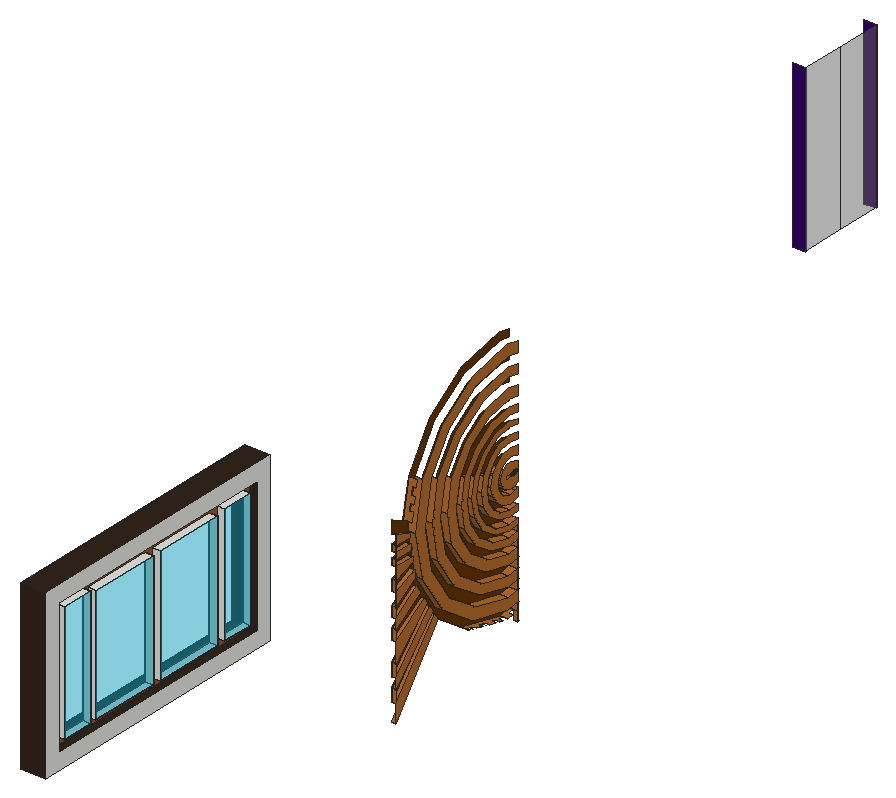
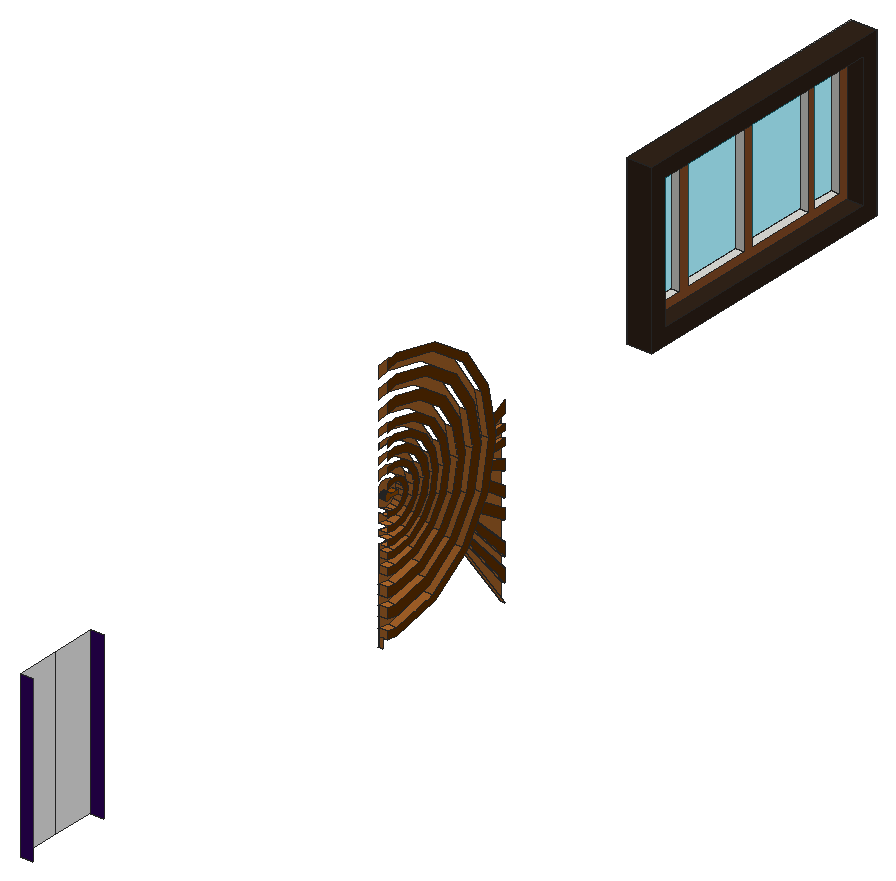
# SketchUp Ruby script. Lengths in inches.
U = 1.inch
M = Sketchup.active_model
def pt(a) = Geom::Point3d.new(a.map { |v| v * U })
def face(e, loops, mat)
  f = e.add_face(loops[0].map { |a| pt(a) })
  loops[1..].each { |l| e.add_face(l.map { |a| pt(a) }).erase! }
  f.material = f.back_material = mat if mat
  f
end
# faces: each face lists its corners as indices into pts; further lists are holes
def faces(e, pts, list, mat = nil) = list.each { |f| face(e, (f[0].is_a?(Array) ? f : [f]).map { |l| l.map { |i| pts[i] } }, mat) }
# xy, xz, yz: faces in a plane at the given z, y or x. An outline is a flat list of corners, or four numbers for a rectangle; further outlines are holes
def ring(l) = l.size == 4 ? [[l[0], l[1]], [l[2], l[1]], [l[2], l[3]], [l[0], l[3]]] : l.each_slice(2).to_a
def flat(e, list, mat, &to3) = list.each { |f| face(e, (f[0].is_a?(Array) ? f : [f]).map { |l| ring(l).map { |u, v| to3.(u, v) } }, mat) }
def xy(e, z, list, mat = nil) = flat(e, list, mat) { |x, y| [x, y, z] }
def xz(e, y, list, mat = nil) = flat(e, list, mat) { |x, z| [x, y, z] }
def yz(e, x, list, mat = nil) = flat(e, list, mat) { |y, z| [x, y, z] }
def lines(e, pts, list) = list.each { |a, b| e.add_line(pt(pts[a]), pt(pts[b])) }
# prism: a flat outline (further loops are holes) pulled along v
def prism(e, loops, v, mat = nil)
  f = face(e, loops, mat); d = Geom::Vector3d.new(v.map { |x| x * U })
  f.pushpull(f.normal.samedirection?(d) ? d.length : -d.length)
end
def box(e, o, s, mat = nil) = prism(e, [[o, [o[0] + s[0], o[1], o[2]], [o[0] + s[0], o[1] + s[1], o[2]], [o[0], o[1] + s[1], o[2]]]], [0, 0, s[2]], mat)
def at(x, y, z, deg = 0) = Geom::Transformation.translation(pt([x, y, z])) * Geom::Transformation.rotation(ORIGIN, Z_AXIS, deg.degrees)
def axes(o, x, y, z) = Geom::Transformation.new([*x, 0, *y, 0, *z, 0, *pt(o).to_a, 1])
def part(name) = M.definitions.add(name)
# library, detail: a bought-in or finely detailed component or shape, given as its bounding box
def library(name, o, s) = part(name).tap { |d| box(d.entities, o, s) }
def detail(e, o, s) = box(e.add_group.entities, o, s)
def put(e, d, t, mat = nil) = e.add_instance(d, t).tap { |i| i.material = mat if mat }
def group(e, t, mat = nil) = e.add_group.tap { |g| g.transformation = t; g.material = mat if mat }.entities
root = M.entities
M.materials.add("Teddy_HairLight").color = [51, 36, 26]
M.materials.add("[Color C07]").color = [153, 76, 0]
M.materials.add("[Color C08]").color = [102, 51, 0]
M.materials.add("[Color J08]").color = [51, 0, 102]
M.materials.add("[Translucent Glass Gray]").color = [128, 128, 128]
M.materials["[Translucent Glass Gray]"].alpha = 0.5
M.materials.add("[Translucent Glass Tinted]").color = [8, 201, 241]
M.materials["[Translucent Glass Tinted]"].alpha = 0.48
M.materials.add("[Wood Bamboo]").color = [177, 105, 43]
M.materials.add("[Wood Cherry Original]").color = [152, 86, 42]
xy(root,163.5,[[205.625,163,206.625,167.79]],"[Wood Bamboo]")
xy(root,165.03,[[205.625,163,206.625,167.5]],"[Wood Bamboo]")
xy(root,166.26,[[203,56.17,209,122.7]],"Teddy_HairLight")
xy(root,166.5625,[[205.625,163,206.625,167.2]],"[Wood Bamboo]")
xy(root,168,[[205.625,163,206.625,166.92]],"[Wood Bamboo]")
xy(root,168.48,[[205.125,195.3125,206.625,197.375]],"[Color C07]")
xy(root,170.08,[[203,59.99,207,118.89]],"Teddy_HairLight")
xy(root,172.08,[[207,61.95,209,69.57],[207,109.39,209,117.01]])
xy(root,172.14,[[207,71.08,209,88.08],[207,90.15,209,107.15]])
xy(root,199.64,[[207,71.08,209,88.08],[207,90.15,209,107.15]])
xy(root,200.2,[[207,61.95,209,69.57],[207,109.39,209,117.01]])
xy(root,201.92,[[203,59.99,207,118.89]],"Teddy_HairLight")
xy(root,205.74,[[203,56.17,209,122.7]],"Teddy_HairLight")
xz(root,56.17,[[203,166.26,209,205.74]],"Teddy_HairLight")
xz(root,59.99,[[203,170.08,207,201.92]],"Teddy_HairLight")
xz(root,61.95,[[207,172.08,209,200.2]])
xz(root,69.57,[[207,172.08,209,200.2]])
xz(root,71.08,[[207,172.14,209,199.64]])
xz(root,88.08,[[207,172.14,209,199.64]])
xz(root,90.15,[[207,172.14,209,199.64]])
xz(root,107.15,[[207,172.14,209,199.64]])
xz(root,109.39,[[207,172.08,209,200.2]])
xz(root,117.01,[[207,172.08,209,200.2]])
xz(root,118.89,[[203,170.08,207,201.92]],"Teddy_HairLight")
xz(root,122.7,[[203,166.26,209,205.74]],"Teddy_HairLight")
xz(root,163,[[205.625,134.4,206.625,137.43],[205.625,139.87,206.625,142.97],[205.625,147.6,206.625,150.15],[205.625,152.47,206.625,154.91],[205.625,158.04,206.625,160.59],
  [205.625,163.5,206.625,165.03],[205.625,166.5625,206.625,168]],"[Wood Bamboo]")
xz(root,195.3125,[[205.125,167.54,206.625,168.48]],"[Wood Bamboo]")
xz(root,198.97,[[205.625,136.14,206.625,138.38],[204.625,138.38,206.625,140.23],[204.625,142.82,206.625,145.13],[204.625,147.33,206.625,149.63],[204.625,151.92,206.625,153.68],
  [204.625,155.31,206.625,156.77]],"[Wood Bamboo]")
xz(root,311.38,[[182,157.72,185,196.65]],"[Color J08]")
xz(root,332.23,[[182,157.72,185,196.65]],"[Color J08]")
yz(root,185,[[311.38,157.72,321.81,196.65],[321.81,157.72,332.23,196.65]],"[Translucent Glass Gray]")
yz(root,203,[[[56.17,166.26,122.7,205.74],[59.99,170.08,118.89,201.92]]],"Teddy_HairLight")
yz(root,204.625,[[196.125,137.91,184.88,140.45,183.75,141.24,175.42,147.03,169.125,156.6875,166.92,168,169.125,179.3125,175.42,188.97,184.88,195.55,196.125,198.09,198.97,197.62,198.97,195.77,196.18,196.23,185.63,193.84,176.76,187.67,170.85,178.61,168.78,168,170.85,157.39,176.76,148.33,185.63,142.16,196.18,139.77,198.97,140.23,198.97,138.38],[196.26,142.37,186.68,144.54,178.62,150.14,173.26,158.36,171.38,168,173.26,177.64,178.62,185.86,186.68,191.46,196.26,193.63,198.97,193.18,198.97,190.87,196.33,191.3,187.62,189.33,180.29,184.24,175.42,176.76,173.71,168,175.42,159.24,180.29,151.76,187.62,146.67,196.33,144.7,198.97,145.13,198.97,142.82],[196.39,146.91,188.51,148.69,181.88,153.3,177.47,160.07,175.92,168,177.47,175.93,181.88,182.7,188.51,187.31,196.39,189.09,198.97,188.67,198.97,186.37,196.46,186.78,189.44,185.2,183.54,181.09,179.6,175.0625,178.23,168,179.6,160.9375,183.54,154.91,189.44,150.8,196.46,149.22,198.97,149.63,198.97,147.33],[196.53,151.52,190.375,152.91,185.19,156.52,181.74,161.8,180.53,168,181.74,174.2,185.19,179.48,190.375,183.09,196.53,184.48,198.97,184.08,198.97,182.32,196.58,182.71,191.08,181.47,186.46,178.25,183.38,173.53,182.3,168,183.38,162.47,186.46,157.75,191.08,154.53,196.58,153.29,198.97,153.68,198.97,151.92],[196.63,154.92,191.75,156.03,187.63,158.89,184.9,163.08,183.9375,168,184.9,172.92,187.63,177.11,191.75,179.97,196.63,181.08,198.97,180.69,198.97,179.23,196.67,179.61,192.34,178.63,188.6875,176.09,186.26,172.36,185.4,168,186.26,163.64,188.6875,159.91,192.34,157.37,196.67,156.39,198.97,156.77,198.97,155.31],
  [196.71,157.66,192.85,158.53,189.59,160.79,187.43,164.11,186.67,168,187.43,171.89,189.59,175.21,192.85,177.47,196.71,178.34,198.98,177.97,198.98,176.35,196.76,176.71,193.51,175.97,190.77,174.07,188.94,171.27,188.31,168,188.94,164.73,190.77,161.93,193.51,160.03,196.76,159.29,198.98,159.65,198.98,158.03],[196.8,160.75,194.09,161.36,191.8125,162.95,190.3,165.27,189.76,168,190.3,170.73,191.8125,173.05,194.09,174.64,196.8,175.25,198.98,174.89,198.98,173.52,196.84,173.875,194.65,173.38,192.8,172.09,191.57,170.21,191.14,168,191.57,165.79,192.8,163.91,194.65,162.62,196.84,162.125,198.98,162.48,198.98,161.11],[196.9,163.99,195.4,164.33,194.14,165.21,193.3,166.49,193.01,168,193.3,169.51,194.14,170.79,195.4,171.67,196.9,172.01,198.42,171.76,198.98,171.41,198.98,170.15,198.03,170.73,196.93,170.91,195.85,170.66,194.93,170.03,194.32,169.09,194.11,168,194.32,166.91,194.93,165.97,195.85,165.34,196.93,165.09,198.03,165.27,198.98,165.85,198.98,164.59,198.42,164.24]],"[Color C08]")
yz(root,205.125,[[198.08,167.4,197.875,167.45,197.68,167.54,197.53,167.68,195.3125,167.54,195.3125,168.48,197.375,168.48,197.47,168.67,197.61,168.83,197.79,168.94,197.99,169.01,198.2,169.02,198.41,168.98,198.6,168.88,198.76,168.74,198.87,168.57,198.9375,168.36,198.95,168.15,198.91,167.94,198.8125,167.76,198.67,167.6,198.49,167.48,198.29,167.41]],"[Color C07]")
yz(root,205.625,[[163,134.4,163,137.43,173.89,149.38,174.54,148.375],[163,139.87,163,142.97,172.24,151.91,173.02,150.72],[163,147.6,163,150.15,170.29,154.9,171.46,153.11],[163,152.47,163,154.91,168.7,158.84,169.125,156.6875],[163,158.04,163,160.59,168.01,162.39,168.36,160.58],
  [163,163.5,163,165.03,167.5,165.03,167.79,163.5],[163,166.5625,163,168,166.92,168,167.2,166.5625],[167.08,168.86,163,170.21,163,173.125,167.48,170.9]],"[Color C08]")
yz(root,206.625,[[163,130.19,163,134.4,174.54,148.375,175.42,147.03],[198.97,136.14,198.98,138.38],[163,137.43,163,139.87,173.02,150.72,173.89,149.38],[198.97,138.38,198.98,140.23],[196.18,139.77,185.63,142.16,176.76,148.33,170.85,157.39,168.78,168,170.85,178.61,176.76,187.67,185.63,193.84,196.18,196.23,198.97,195.77,198.97,193.18,196.26,193.63,186.68,191.46,178.62,185.86,173.26,177.64,171.38,168,173.26,158.36,178.62,150.14,186.68,144.54,196.26,142.37,198.97,142.82,198.97,140.23],
  [198.97,140.23,198.98,142.82],[198.97,142.82,198.97,145.13,198.98,145.14,198.98,142.82],[163,142.97,163,147.6,171.46,153.11,172.24,151.91],[196.33,144.7,187.62,146.67,180.29,151.76,175.42,159.24,173.71,168,175.42,176.76,180.29,184.24,187.62,189.33,196.33,191.3,198.97,190.87,198.97,188.67,196.39,189.09,188.51,187.31,181.88,182.7,177.47,175.93,175.92,168,177.47,160.07,181.88,153.3,188.51,148.69,196.39,146.91,198.97,147.33,198.97,145.13],[198.97,145.13,198.97,147.33,198.98,147.34,198.98,145.14],
  [198.97,147.33,198.97,149.63,198.98,149.63,198.98,147.34],[196.46,149.22,189.44,150.8,183.54,154.91,179.6,160.9375,178.23,168,179.6,175.0625,183.54,181.09,189.44,185.2,196.46,186.78,198.97,186.37,198.97,184.08,196.53,184.48,190.375,183.09,185.19,179.48,181.74,174.2,180.53,168,181.74,161.8,185.19,156.52,190.375,152.91,196.53,151.52,198.97,151.92,198.97,149.63],[198.97,149.63,198.98,151.92],[163,150.15,163,152.47,169.125,156.6875,170.29,154.9],[198.97,151.92,198.98,153.68],
  [196.58,153.29,191.08,154.53,186.46,157.75,183.38,162.47,182.3,168,183.38,173.53,186.46,178.25,191.08,181.47,196.58,182.71,198.97,182.32,198.97,180.69,196.63,181.08,191.75,179.97,187.63,177.11,184.9,172.92,183.9375,168,184.9,163.08,187.63,158.89,191.75,156.03,196.63,154.92,198.97,155.31,198.97,153.68],[198.97,153.68,198.97,155.31,198.98,155.3125,198.98,153.68],[162.98,154.9,162.98,158.03,163,158.04,163,154.91],[163,154.91,163,158.04,168.36,160.58,168.7,158.84],[198.97,155.31,198.97,156.77,198.98,156.77,198.98,155.3125],
  [196.67,156.39,192.34,157.37,188.6875,159.91,186.26,163.64,185.4,168,186.26,172.36,188.6875,176.09,192.34,178.63,196.67,179.61,198.97,179.23,198.97,177.99,196.71,178.36,192.84,177.49,189.58,175.22,187.41,171.9,186.65,168,187.41,164.1,189.58,160.78,192.84,158.51,196.71,157.64,198.97,158.01,198.97,156.77],[198.97,156.77,198.97,158.01,196.71,157.64,192.84,158.51,189.58,160.78,187.41,164.1,186.65,168,187.41,171.9,189.58,175.22,192.84,177.49,196.71,178.36,198.97,177.99,198.97,179.23,198.98,179.23,198.98,177.97,196.71,178.34,192.85,177.47,189.59,175.21,187.43,171.89,186.67,168,187.43,164.11,189.59,160.79,192.85,158.53,196.71,157.66,198.98,158.03,198.98,156.77],[162.98,158.03,162.98,160.58,163,160.59,163,158.04],[196.76,159.29,193.51,160.03,190.77,161.93,188.94,164.73,188.31,168,188.94,171.27,190.77,174.07,193.51,175.97,196.76,176.71,198.98,176.35,198.98,174.89,196.8,175.25,194.09,174.64,191.8125,173.05,190.3,170.73,189.76,168,190.3,165.27,191.8125,162.95,194.09,161.36,196.8,160.75,198.98,161.11,198.98,159.65],[162.98,160.58,162.98,168,163,168,163,160.59],
  [163,160.59,163,163.5,167.79,163.5,168.01,162.39],[196.84,162.125,194.65,162.62,192.8,163.91,191.57,165.79,191.14,168,191.57,170.21,192.8,172.09,194.65,173.38,196.84,173.875,198.98,173.52,198.98,171.41,198.42,171.76,196.9,172.01,195.4,171.67,194.14,170.79,193.3,169.51,193.01,168,193.3,166.49,194.14,165.21,195.4,164.33,196.9,163.99,198.42,164.24,198.98,164.59,198.98,162.48],[163,165.03,163,166.5625,167.2,166.5625,167.5,165.03],[[196.93,165.09,195.85,165.34,194.93,165.97,194.32,166.91,194.11,168,194.32,169.09,194.93,170.03,195.85,170.66,196.93,170.91,198.03,170.73,198.98,170.15,198.98,165.85,198.03,165.27],[198.08,167.4,198.29,167.41,198.49,167.48,198.67,167.6,198.8125,167.76,198.91,167.94,198.95,168.15,198.9375,168.36,198.87,168.57,198.76,168.74,198.6,168.88,198.41,168.98,198.2,169.02,197.99,169.01,197.79,168.94,197.61,168.83,197.47,168.67,197.375,168.48,195.3125,168.48,195.3125,167.54,197.53,167.68,197.68,167.54,197.875,167.45]],[162.98,168,162.98,170.22,163,170.21,163,168],
  [163,168,163,170.21,167.08,168.86,166.92,168]],"[Wood Bamboo]")
yz(root,207,[[[59.99,170.08,118.89,201.92],[90.15,172.14,107.15,199.64],[71.08,172.14,88.08,199.64],[109.39,172.08,117.01,200.2],[61.95,172.08,69.57,200.2]]],"[Wood Cherry Original]")
yz(root,209,[[[56.17,166.26,122.7,205.74],[59.99,170.08,118.89,201.92]]])
yz(root,209,[[61.95,172.08,69.57,200.2],[109.39,172.08,117.01,200.2],[71.08,172.14,88.08,199.64],[90.15,172.14,107.15,199.64]],"[Translucent Glass Tinted]")
p = [[206.625,163,130.19],[206.625,175.42,147.03],[205.625,175.42,147.03],[205.625,163,130.19],[206.625,174.54,148.375],[206.625,163,134.4],
  [205.625,163,134.4],[205.625,174.54,148.375],[206.625,163,137.43],[206.625,173.89,149.38],[205.625,173.89,149.38],[205.625,163,137.43],
  [204.625,196.125,137.91],[205.625,196.125,137.91],[205.625,194.52,138.27],[206.625,194.52,138.27],[206.625,193.55,138.49],[205.625,193.55,138.49],
  [205.625,192.59,138.71],[206.625,192.59,138.71],[206.625,191.625,138.93],[206.625,190.66,139.15],[205.625,190.66,139.15],[205.625,189.7,139.36],
  [205.625,188.74,139.58],[205.625,188.25,139.69],[206.625,188.25,139.69],[206.625,187.77,139.8],[206.625,186.81,140.02],[205.625,186.81,140.02],
  [205.625,185.85,140.23],[205.625,184.88,140.45],[204.625,184.88,140.45],[204.625,198.97,138.38],[205.625,198.97,138.38],[205.625,197.55,138.14],
  [206.625,197.55,138.14],[206.625,196.125,137.91],[206.625,185.63,142.16],[206.625,196.18,139.77],[204.625,196.18,139.77],[204.625,185.63,142.16],
  [206.625,198.97,140.23],[204.625,198.97,140.23],[206.625,173.02,150.72],[206.625,163,139.87],[205.625,163,139.87],[205.625,173.02,150.72],
  [206.625,184.88,140.45],[206.625,184.02,141.05],[205.625,184.02,141.05],[205.625,183.08,141.7],[206.625,183.08,141.7],[206.625,182.1875,142.33],
  [205.625,182.1875,142.33],[205.625,181.2,143.02],[206.625,181.2,143.02],[206.625,179.7,144.06],[205.5,179.7,144.06],[205.5,178.05,145.21],
  [206.625,178.05,145.21],[206.625,176.73,146.12],[205.625,176.73,146.12],[204.625,175.42,147.03],[204.625,183.75,141.24],[206.625,176.76,148.33],
  [204.625,176.76,148.33],[206.625,196.26,142.37],[206.625,186.68,144.54],[204.625,186.68,144.54],[204.625,196.26,142.37],[206.625,198.97,142.82],
  [204.625,198.97,142.82],[206.625,163,142.97],[206.625,172.24,151.91],[205.625,172.24,151.91],[205.625,163,142.97],[206.625,178.62,150.14],
  [204.625,178.62,150.14],[206.625,187.62,146.67],[206.625,196.33,144.7],[204.625,196.33,144.7],[204.625,187.62,146.67],[206.625,198.97,145.13],
  [204.625,198.97,145.13],[206.625,180.29,151.76],[204.625,180.29,151.76],[206.625,196.39,146.91],[206.625,188.51,148.69],[204.625,188.51,148.69],
  [204.625,196.39,146.91],[206.625,198.97,147.33],[204.625,198.97,147.33],[206.625,171.46,153.11],[205.625,171.46,153.11],[205.625,170.29,154.9],
  [206.625,170.29,154.9],[206.625,169.125,156.6875],[205.625,169.125,156.6875],[204.625,169.125,156.6875],[206.625,163,147.6],[205.625,163,147.6],
  [206.625,170.85,157.39],[204.625,170.85,157.39],[206.625,181.88,153.3],[204.625,181.88,153.3],[206.625,189.44,150.8],[206.625,196.46,149.22],
  [204.625,196.46,149.22],[204.625,189.44,150.8],[206.625,198.97,149.63],[204.625,198.97,149.63],[206.625,163,150.15],[205.625,163,150.15],
  [206.625,173.26,158.36],[204.625,173.26,158.36],[206.625,183.54,154.91],[204.625,183.54,154.91],[206.625,196.53,151.52],[206.625,190.375,152.91],
  [204.625,190.375,152.91],[204.625,196.53,151.52],[206.625,198.97,151.92],[204.625,198.97,151.92],[206.625,175.42,159.24],[204.625,175.42,159.24],
  [206.625,163,152.47],[205.625,163,152.47],[206.625,185.19,156.52],[204.625,185.19,156.52],[206.625,177.47,160.07],[204.625,177.47,160.07],
  [206.625,191.08,154.53],[206.625,196.58,153.29],[204.625,196.58,153.29],[204.625,191.08,154.53],[206.625,198.97,153.68],[204.625,198.97,153.68],
  [206.625,186.46,157.75],[204.625,186.46,157.75],[206.625,163,154.91],[206.625,168.7,158.84],[205.625,168.7,158.84],[205.625,163,154.91],
  [206.625,179.6,160.9375],[204.625,179.6,160.9375],[206.625,196.63,154.92],[206.625,191.75,156.03],[204.625,191.75,156.03],[204.625,196.63,154.92],
  [206.625,198.97,155.31],[204.625,198.97,155.31],[206.625,187.63,158.89],[204.625,187.63,158.89],[206.625,192.34,157.37],[206.625,196.67,156.39],
  [204.625,196.67,156.39],[204.625,192.34,157.37],[206.625,198.97,156.77],[204.625,198.97,156.77],[206.625,181.74,161.8],[204.625,181.74,161.8],
  [206.625,168.36,160.58],[205.625,168.36,160.58],[205.625,168.01,162.39],[206.625,168.01,162.39],[206.625,167.79,163.5],[205.625,167.79,163.5],
  [205.625,167.5,165.03],[206.625,167.5,165.03],[206.625,167.2,166.5625],[205.625,167.2,166.5625],[205.625,166.92,168],[204.625,166.92,168],
  [206.625,168.78,168],[204.625,168.78,168],[206.625,188.6875,159.91],[204.625,188.6875,159.91],[206.625,183.38,162.47],[204.625,183.38,162.47],
  [206.625,196.71,157.66],[206.625,192.85,158.53],[204.625,192.85,158.53],[204.625,196.71,157.66],[206.625,198.98,158.03],[204.625,198.98,158.03],
  [206.625,163,158.04],[205.625,163,158.04],[206.625,171.38,168],[204.625,171.38,168],[206.625,189.59,160.79],[204.625,189.59,160.79],
  [206.625,184.9,163.08],[204.625,184.9,163.08],[206.625,173.71,168],[204.625,173.71,168],[206.625,193.51,160.03],[206.625,196.76,159.29],
  [204.625,196.76,159.29],[204.625,193.51,160.03],[206.625,198.98,159.65],[204.625,198.98,159.65],[206.625,186.26,163.64],[204.625,186.26,163.64],
  [206.625,190.77,161.93],[204.625,190.77,161.93],[206.625,175.92,168],[204.625,175.92,168],[206.625,163,160.59],[205.625,163,160.59],
  [206.625,196.8,160.75],[206.625,194.09,161.36],[204.625,194.09,161.36],[204.625,196.8,160.75],[206.625,198.98,161.11],[204.625,198.98,161.11],
  [206.625,187.43,164.11],[204.625,187.43,164.11],[206.625,178.23,168],[204.625,178.23,168],[206.625,191.8125,162.95],[204.625,191.8125,162.95],
  [206.625,180.53,168],[204.625,180.53,168],[206.625,188.94,164.73],[204.625,188.94,164.73],[206.625,194.65,162.62],[206.625,196.84,162.125],
  [204.625,196.84,162.125],[204.625,194.65,162.62],[206.625,198.98,162.48],[204.625,198.98,162.48],[206.625,182.3,168],[204.625,182.3,168],
  [206.625,192.8,163.91],[204.625,192.8,163.91],[206.625,190.3,165.27],[204.625,190.3,165.27],[206.625,183.9375,168],[204.625,183.9375,168],
  [206.625,185.4,168],[204.625,185.4,168],[206.625,191.57,165.79],[204.625,191.57,165.79],[206.625,196.9,163.99],[206.625,195.4,164.33],
  [204.625,195.4,164.33],[204.625,196.9,163.99],[206.625,198.42,164.24],[204.625,198.42,164.24],[206.625,186.67,168],[204.625,186.67,168],
  [206.625,198.98,164.59],[204.625,198.98,164.59],[206.625,194.14,165.21],[204.625,194.14,165.21],[206.625,188.31,168],[204.625,188.31,168],
  [206.625,195.85,165.34],[206.625,196.93,165.09],[204.625,196.93,165.09],[204.625,195.85,165.34],[206.625,198.03,165.27],[204.625,198.03,165.27],
  [206.625,193.3,166.49],[204.625,193.3,166.49],[206.625,189.76,168],[204.625,189.76,168],[206.625,194.93,165.97],[204.625,194.93,165.97],
  [206.625,198.98,165.85],[204.625,198.98,165.85],[206.625,191.14,168],[204.625,191.14,168],[206.625,194.32,166.91],[204.625,194.32,166.91],
  [206.625,193.01,168],[204.625,193.01,168],[206.625,194.11,168],[204.625,194.11,168],[206.625,197.875,167.45],[206.625,197.68,167.54],
  [205.125,197.68,167.54],[205.125,197.875,167.45],[206.625,198.08,167.4],[205.125,198.08,167.4],[206.625,198.29,167.41],[205.125,198.29,167.41],
  [206.625,198.49,167.48],[205.125,198.49,167.48],[206.625,197.53,167.68],[206.625,195.3125,167.54],[205.125,195.3125,167.54],[205.125,197.53,167.68],
  [206.625,198.67,167.6],[205.125,198.67,167.6],[206.625,198.8125,167.76],[205.125,198.8125,167.76],[206.625,198.91,167.94],[205.125,198.91,167.94],
  [206.625,198.95,168.15],[205.125,198.95,168.15],[206.625,166.92,168],[206.625,167.08,168.86],[205.625,167.08,168.86],[205.625,167.48,170.9],
  [206.625,167.48,170.9],[206.625,167.88,172.94],[205.625,167.88,172.94],[205.625,168.17,174.44],[206.625,168.17,174.44],[206.625,168.49,176.05],
  [205.625,168.49,176.05],[205.625,168.83,177.79],[206.625,168.83,177.79],[206.625,169.125,179.3125],[205.625,169.125,179.3125],[204.625,169.125,179.3125],
  [206.625,170.85,178.61],[204.625,170.85,178.61],[206.625,173.26,177.64],[204.625,173.26,177.64],[206.625,175.42,176.76],[204.625,175.42,176.76],
  [206.625,177.47,175.93],[204.625,177.47,175.93],[206.625,179.6,175.0625],[204.625,179.6,175.0625],[206.625,181.74,174.2],[204.625,181.74,174.2],
  [206.625,183.38,173.53],[204.625,183.38,173.53],[206.625,184.9,172.92],[204.625,184.9,172.92],[206.625,186.26,172.36],[204.625,186.26,172.36],
  [206.625,187.43,171.89],[204.625,187.43,171.89],[206.625,188.94,171.27],[204.625,188.94,171.27],[206.625,190.3,170.73],[204.625,190.3,170.73],
  [206.625,191.57,170.21],[204.625,191.57,170.21],[206.625,193.3,169.51],[204.625,193.3,169.51],[206.625,194.32,169.09],[204.625,194.32,169.09],
  [206.625,198.9375,168.36],[205.125,198.9375,168.36],[206.625,198.87,168.57],[205.125,198.87,168.57],[206.625,197.375,168.48],[206.625,197.47,168.67],
  [205.125,197.47,168.67],[205.125,197.375,168.48],[206.625,198.76,168.74],[205.125,198.76,168.74],[206.625,197.61,168.83],[205.125,197.61,168.83],
  [206.625,198.6,168.88],[205.125,198.6,168.88],[206.625,197.79,168.94],[205.125,197.79,168.94],[206.625,163,170.21],[205.625,163,170.21],
  [206.625,197.99,169.01],[205.125,197.99,169.01],[206.625,198.41,168.98],[205.125,198.41,168.98],[206.625,198.2,169.02],[205.125,198.2,169.02],
  [206.625,194.93,170.03],[204.625,194.93,170.03],[206.625,194.14,170.79],[204.625,194.14,170.79],[206.625,199.1875,156.8],[206.625,198.98,156.77],
  [206.625,199.2,155.35],[206.625,198.98,155.3125],[206.625,199.23,153.72],[206.625,198.98,153.68],[206.625,199.25,151.97],[206.625,198.98,151.92],
  [206.625,199.33,149.6875],[206.625,198.98,149.63],[206.625,199.33,147.39],[206.625,198.98,147.34],[206.625,199.32,145.19],[206.625,198.98,145.14],
  [206.625,199.34,142.88],[206.625,198.98,142.82],[206.625,199.38,140.3],[206.625,198.98,140.23],[206.625,199.26,138.43],[206.625,198.98,138.38],
  [206.625,199.33,136.2],[206.625,198.98,136.14],[206.625,189.7,139.36],[206.625,188.74,139.58],[206.625,185.85,140.23]]
faces(root,p,[[0,1,2,3],[4,5,6,7],[8,9,10,11],[12,13,14,15,16,17,18,19,20,21,22,23,24,25,26,27,28,29,30,31,32],[33,34,35,36,37,13,12],[38,39,40,41],[39,42,43,40],[44,45,46,47],
  [48,49,50,51,52,53,54,55,56,57,58,59,60,61,62,2,63,64,32,31],[65,38,41,66],[67,68,69,70],[71,67,70,72],[73,74,75,76],[68,77,78,69],[79,80,81,82],[80,83,84,81],
  [85,79,82,86],[87,88,89,90],[91,87,90,92],[1,4,7,10,9,44,47,75,74,93,94,95,96,97,98,99,63,2],[93,100,101,94],[102,65,66,103],[88,104,105,89],[106,107,108,109],
  [107,110,111,108],[112,96,95,113],[77,114,115,78],[116,106,109,117],[118,119,120,121],[122,118,121,123],[124,85,86,125],[97,126,127,98],
  [119,128,129,120],[104,130,131,105],[132,133,134,135],[133,136,137,134],[138,132,135,139],[140,141,142,143],[144,116,117,145],[146,147,148,149],
  [150,146,149,151],[147,152,153,148],[154,155,156,157],[155,158,159,156],[128,160,161,129],[99,98,142,141,162,163,164,165,166,167,168,169,170,171,172,173],[174,102,103,175],[176,154,157,177],
  [178,138,139,179],[180,181,182,183],[184,180,183,185],[162,186,187,163],[114,188,189,115],[181,190,191,182],[152,192,193,153],[194,124,125,195],
  [196,197,198,199],[197,200,201,198],[202,176,177,203],[204,196,199,205],[130,206,207,131],[208,165,164,209],[210,211,212,213],[214,210,213,215],
  [190,216,217,191],[218,144,145,219],[211,220,221,212],[160,222,223,161],[224,204,205,225],[226,227,228,229],[227,230,231,228],[232,178,179,233],
  [234,226,229,235],[220,236,237,221],[192,238,239,193],[240,202,203,241],[242,234,235,243],[244,245,246,247],[248,244,247,249],[216,250,251,217],
  [252,248,249,253],[245,254,255,246],[256,224,225,257],[258,259,260,261],[259,262,263,260],[254,264,265,255],[236,266,267,237],[268,258,261,269],
  [262,270,271,263],[272,242,243,273],[274,268,269,275],[264,276,277,265],[278,274,275,279],[302,303,304,305,306,307,308,309,310,311,312,313,314,315,316,317,173,172],[318,174,175,319],[188,320,321,189],
  [322,194,195,323],[206,324,325,207],[326,218,219,327],[222,328,329,223],[330,232,233,331],[238,332,333,239],[334,240,241,335],[250,336,337,251],
  [338,256,257,339],[266,340,341,267],[342,272,273,343],[276,344,345,277],[346,278,279,347],[303,364,365,304],[372,346,347,373],[344,374,375,345]],"[Wood Bamboo]")
faces(root,p,[[280,281,282,283],[284,280,283,285],[286,284,285,287],[288,286,287,289],[290,291,292,293],[281,290,293,282],[294,288,289,295],[296,294,295,297],
  [298,296,297,299],[300,298,299,301],[348,300,301,349],[350,348,349,351],[352,353,354,355],[356,350,351,357],[353,358,359,354],[360,356,357,361],
  [358,362,363,359],[362,366,367,363],[368,360,361,369],[366,370,371,367],[370,368,369,371]],"[Color C07]")
lines(root,p,[[376,377],[378,379],[380,381],[382,383],[384,385],[386,387],[388,389],[390,391],[392,393],[394,395],[396,397],[398,23],
  [399,24],[400,30]])
